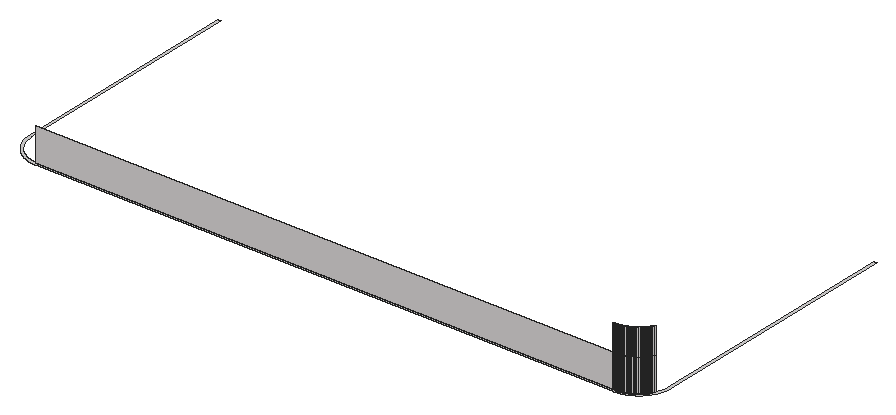
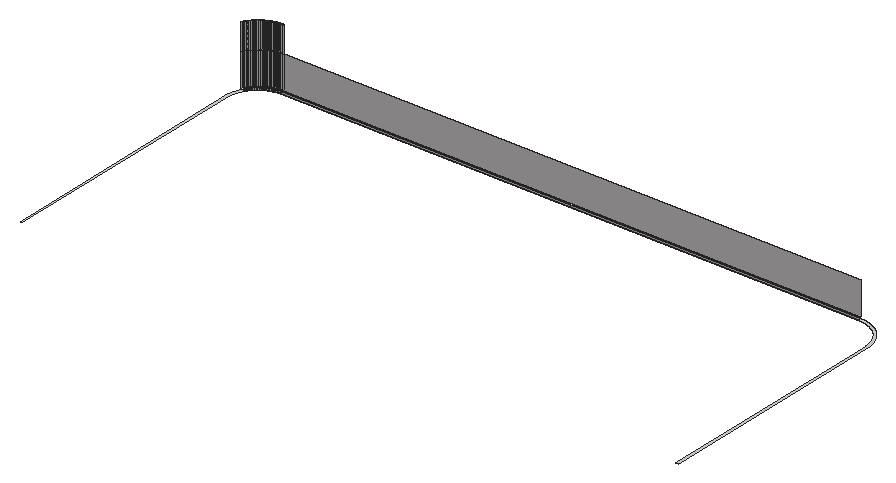
# SketchUp Ruby script. Lengths in inches.
U = 1.inch
M = Sketchup.active_model
def pt(a) = Geom::Point3d.new(a.map { |v| v * U })
def face(e, loops, mat)
  f = e.add_face(loops[0].map { |a| pt(a) })
  loops[1..].each { |l| e.add_face(l.map { |a| pt(a) }).erase! }
  f.material = f.back_material = mat if mat
  f
end
# faces: each face lists its corners as indices into pts; further lists are holes
def faces(e, pts, list, mat = nil) = list.each { |f| face(e, (f[0].is_a?(Array) ? f : [f]).map { |l| l.map { |i| pts[i] } }, mat) }
# xy, xz, yz: faces in a plane at the given z, y or x. An outline is a flat list of corners, or four numbers for a rectangle; further outlines are holes
def ring(l) = l.size == 4 ? [[l[0], l[1]], [l[2], l[1]], [l[2], l[3]], [l[0], l[3]]] : l.each_slice(2).to_a
def flat(e, list, mat, &to3) = list.each { |f| face(e, (f[0].is_a?(Array) ? f : [f]).map { |l| ring(l).map { |u, v| to3.(u, v) } }, mat) }
def xy(e, z, list, mat = nil) = flat(e, list, mat) { |x, y| [x, y, z] }
def xz(e, y, list, mat = nil) = flat(e, list, mat) { |x, z| [x, y, z] }
def yz(e, x, list, mat = nil) = flat(e, list, mat) { |y, z| [x, y, z] }
def lines(e, pts, list) = list.each { |a, b| e.add_line(pt(pts[a]), pt(pts[b])) }
# prism: a flat outline (further loops are holes) pulled along v
def prism(e, loops, v, mat = nil)
  f = face(e, loops, mat); d = Geom::Vector3d.new(v.map { |x| x * U })
  f.pushpull(f.normal.samedirection?(d) ? d.length : -d.length)
end
def box(e, o, s, mat = nil) = prism(e, [[o, [o[0] + s[0], o[1], o[2]], [o[0] + s[0], o[1] + s[1], o[2]], [o[0], o[1] + s[1], o[2]]]], [0, 0, s[2]], mat)
def at(x, y, z, deg = 0) = Geom::Transformation.translation(pt([x, y, z])) * Geom::Transformation.rotation(ORIGIN, Z_AXIS, deg.degrees)
def axes(o, x, y, z) = Geom::Transformation.new([*x, 0, *y, 0, *z, 0, *pt(o).to_a, 1])
def part(name) = M.definitions.add(name)
# library, detail: a bought-in or finely detailed component or shape, given as its bounding box
def library(name, o, s) = part(name).tap { |d| box(d.entities, o, s) }
def detail(e, o, s) = box(e.add_group.entities, o, s)
def put(e, d, t, mat = nil) = e.add_instance(d, t).tap { |i| i.material = mat if mat }
def group(e, t, mat = nil) = e.add_group.tap { |g| g.transformation = t; g.material = mat if mat }.entities
root = M.entities
M.materials.add("[Quartz Light Brown]").color = [215, 212, 212]
xy(root,368,[[215.8,143,480.2,143,480.39,143.01,480.59,143.01,480.79,143.02,480.98,143.03,481.18,143.05,481.37,143.0625,481.57,143.08,481.76,143.1,481.96,143.13,482.15,143.16,482.35,143.18,482.54,143.22,482.73,143.25,482.93,143.29,483.5,143.41,483.88,143.51,484.07,143.5625,484.26,143.62,484.45,143.67,484.64,143.73,484.82,143.8,485.01,143.86,485.19,143.93,485.56,144.07,485.74,144.14,486.46,144.46,486.63,144.55,486.81,144.63,486.98,144.73,487.16,144.82,487.33,144.91,487.84,145.21,488,145.3125,488.17,145.42,488.33,145.53,488.5,145.64,488.82,145.86,488.97,145.98,489.29,146.22,489.44,146.34,489.59,146.47,489.74,146.59,490.04,146.85,490.18,146.99,490.33,147.12,490.47,147.26,490.61,147.39,490.74,147.53,490.88,147.67,491.01,147.82,491.15,147.96,491.41,148.26,491.53,148.41,491.66,148.56,491.78,148.71,492.02,149.03,492.14,149.18,492.36,149.5,492.47,149.67,492.58,149.83,492.6875,150,492.79,150.16,493.09,150.67,493.18,150.84,493.27,151.02,493.37,151.19,493.45,151.37,493.54,151.54,493.86,152.26,493.93,152.44,494.07,152.81,494.14,152.99,494.2,153.18,494.27,153.36,494.33,153.55,494.38,153.74,494.4375,153.93,494.49,154.12,494.59,154.5,494.71,155.07,494.75,155.27,494.78,155.46,494.82,155.65,494.84,155.85,494.87,156.04,494.9,156.24,494.92,156.43,494.9375,156.63,494.95,156.82,494.97,157.02,494.98,157.21,494.99,157.41,494.99,157.61,495,157.8,495,275,494,275,494,157.63,493.98,157.27,493.97,157.08,493.96,156.9,493.92,156.54,493.9,156.35,493.86,155.99,493.77,155.45,493.57,154.55,493.47,154.2,493.42,154.02,493.37,153.85,493.31,153.67,493.26,153.5,493.2,153.33,493.13,153.15,493.07,152.98,493,152.8125,492.93,152.64,492.86,152.47,492.79,152.31,492.71,152.14,492.64,151.97,492.56,151.81,492.47,151.64,492.39,151.48,492.21,151.16,492.125,151,492.03,150.84,491.9375,150.69,491.84,150.53,491.64,150.22,491.54,150.07,491.43,149.92,491.33,149.77,491.11,149.48,490.99,149.33,490.88,149.19,490.76,149.05,490.65,148.91,490.53,148.77,490.4,148.63,490.28,148.5,490.16,148.36,489.64,147.84,489.5,147.72,489.37,147.6,489.23,147.47,489.09,147.35,488.95,147.24,488.81,147.12,488.67,147.01,488.52,146.89,488.23,146.67,488.08,146.57,487.93,146.46,487.78,146.36,487.47,146.16,487.31,146.0625,487.16,145.97,487,145.875,486.84,145.79,486.52,145.61,486.36,145.53,486.19,145.44,486.03,145.36,485.86,145.29,485.69,145.21,485.53,145.14,485.36,145.07,485.1875,145,485.02,144.93,484.85,144.87,484.67,144.8,484.5,144.74,484.33,144.69,484.15,144.63,483.98,144.58,483.8,144.53,483.45,144.43,482.55,144.23,482.01,144.14,481.65,144.1,481.46,144.08,481.1,144.04,480.92,144.03,480.73,144.02,480.37,144,215.63,144,215.27,144.02,215.08,144.03,214.9,144.04,214.54,144.08,214.35,144.1,213.99,144.14,213.45,144.23,212.55,144.43,212.2,144.53,212.02,144.58,211.85,144.63,211.67,144.69,211.5,144.74,211.33,144.8,211.15,144.87,210.98,144.93,210.8125,145,210.64,145.07,210.47,145.14,210.31,145.21,210.14,145.29,209.97,145.36,209.81,145.44,209.64,145.53,209.48,145.61,209.16,145.79,209,145.875,208.84,145.97,208.69,146.0625,208.53,146.16,208.22,146.36,208.07,146.46,207.92,146.57,207.77,146.67,207.48,146.89,207.33,147.01,207.19,147.12,207.05,147.24,206.91,147.35,206.77,147.47,206.63,147.6,206.5,147.72,206.36,147.84,205.84,148.36,205.72,148.5,205.6,148.63,205.47,148.77,205.35,148.91,205.24,149.05,205.12,149.19,205.01,149.33,204.89,149.48,204.67,149.77,204.57,149.92,204.46,150.07,204.36,150.22,204.16,150.53,204.0625,150.69,203.97,150.84,203.875,151,203.79,151.16,203.61,151.48,203.53,151.64,203.44,151.81,203.36,151.97,203.29,152.14,203.21,152.31,203.14,152.47,203.07,152.64,203,152.8125,202.93,152.98,202.87,153.15,202.8,153.33,202.74,153.5,202.69,153.67,202.63,153.85,202.58,154.02,202.53,154.2,202.43,154.55,202.23,155.45,202.14,155.99,202.1,156.35,202.08,156.54,202.04,156.9,202.03,157.08,202.02,157.27,202,157.63,202,266,201,266,201,157.8,201.01,157.61,201.01,157.41,201.02,157.21,201.03,157.02,201.05,156.82,201.0625,156.63,201.08,156.43,201.1,156.24,201.13,156.04,201.16,155.85,201.18,155.65,201.22,155.46,201.25,155.27,201.29,155.07,201.41,154.5,201.51,154.12,201.5625,153.93,201.62,153.74,201.67,153.55,201.73,153.36,201.8,153.18,201.86,152.99,201.93,152.81,202.07,152.44,202.14,152.26,202.46,151.54,202.55,151.37,202.63,151.19,202.73,151.02,202.82,150.84,202.91,150.67,203.21,150.16,203.3125,150,203.42,149.83,203.53,149.67,203.64,149.5,203.86,149.18,203.98,149.03,204.22,148.71,204.34,148.56,204.47,148.41,204.59,148.26,204.85,147.96,204.99,147.82,205.12,147.67,205.26,147.53,205.39,147.39,205.53,147.26,205.67,147.12,205.82,146.99,205.96,146.85,206.26,146.59,206.41,146.47,206.56,146.34,206.71,146.22,207.03,145.98,207.18,145.86,207.5,145.64,207.67,145.53,207.83,145.42,208,145.3125,208.16,145.21,208.67,144.91,208.84,144.82,209.02,144.73,209.19,144.63,209.37,144.55,209.54,144.46,210.26,144.14,210.44,144.07,210.81,143.93,210.99,143.86,211.18,143.8,211.36,143.73,211.55,143.67,211.74,143.62,211.93,143.5625,212.12,143.51,212.5,143.41,213.07,143.29,213.27,143.25,213.46,143.22,213.65,143.18,213.85,143.16,214.04,143.13,214.24,143.1,214.43,143.08,214.63,143.0625,214.82,143.05,215.02,143.03,215.21,143.02,215.41,143.01,215.61,143.01]],"[Quartz Light Brown]")
xz(root,143,[[216,369,480,384],[480,369,480.2,384],[480,384,480.2,396]],"[Quartz Light Brown]")
xz(root,143.01,[[480.39,369,480.59,384],[480.39,384,480.59,396]],"[Quartz Light Brown]")
xz(root,144,[[216,368,480,369],[480,368,480.18,369],[480.18,368,480.37,369]],"[Quartz Light Brown]")
p = [[480.37,144,369],[480.37,144,368],[480.55,144.01,368],[480.55,144.01,369],[480.73,144.02,368],[480.73,144.02,369],
  [480.92,144.03,368],[480.92,144.03,369],[481.1,144.04,368],[481.1,144.04,369],[481.28,144.06,368],[481.28,144.06,369],
  [481.46,144.08,368],[481.46,144.08,369],[481.65,144.1,368],[481.65,144.1,369],[481.83,144.12,368],[481.83,144.12,369],
  [482.01,144.14,368],[482.01,144.14,369],[482.19,144.17,368],[482.19,144.17,369],[482.37,144.2,368],[482.37,144.2,369],
  [482.55,144.23,368],[482.55,144.23,369],[482.73,144.27,368],[482.73,144.27,369],[482.91,144.31,368],[482.91,144.31,369],
  [483.09,144.35,368],[483.09,144.35,369],[483.27,144.39,368],[483.27,144.39,369],[483.45,144.43,368],[483.45,144.43,369],
  [483.625,144.48,368],[483.625,144.48,369],[483.8,144.53,368],[483.8,144.53,369],[483.98,144.58,368],[483.98,144.58,369],
  [484.15,144.63,368],[484.15,144.63,369],[484.33,144.69,368],[484.33,144.69,369],[484.5,144.74,368],[484.5,144.74,369],
  [484.67,144.8,368],[484.67,144.8,369],[484.85,144.87,368],[484.85,144.87,369],[485.02,144.93,368],[485.02,144.93,369],
  [485.1875,145,368],[485.1875,145,369],[485.36,145.07,368],[485.36,145.07,369],[485.53,145.14,368],[485.53,145.14,369],
  [485.69,145.21,368],[485.69,145.21,369],[485.86,145.29,368],[485.86,145.29,369],[486.03,145.36,368],[486.03,145.36,369],
  [486.19,145.44,368],[486.19,145.44,369],[486.36,145.53,368],[486.36,145.53,369],[486.52,145.61,368],[486.52,145.61,369],
  [486.68,145.7,368],[486.68,145.7,369],[486.84,145.79,368],[486.84,145.79,369],[487,145.875,368],[487,145.875,369],
  [487.16,145.97,368],[487.16,145.97,369],[487.31,146.0625,368],[487.31,146.0625,369],[487.47,146.16,368],[487.47,146.16,369],
  [487.625,146.26,368],[487.625,146.26,369],[487.78,146.36,368],[487.78,146.36,369],[487.93,146.46,368],[487.93,146.46,369],
  [488.08,146.57,368],[488.08,146.57,369],[488.23,146.67,368],[488.23,146.67,369],[488.375,146.78,368],[488.375,146.78,369],
  [488.52,146.89,368],[488.52,146.89,369],[488.67,147.01,368],[488.67,147.01,369],[488.81,147.12,368],[488.81,147.12,369],
  [488.95,147.24,368],[488.95,147.24,369],[489.09,147.35,368],[489.09,147.35,369],[489.23,147.47,368],[489.23,147.47,369],
  [489.37,147.6,368],[489.37,147.6,369],[489.5,147.72,368],[489.5,147.72,369],[489.64,147.84,368],[489.64,147.84,369],
  [489.77,147.97,368],[489.77,147.97,369],[489.9,148.1,368],[489.9,148.1,369],[490.03,148.23,368],[490.03,148.23,369],
  [490.16,148.36,368],[490.16,148.36,369],[490.28,148.5,368],[490.28,148.5,369],[490.4,148.63,368],[490.4,148.63,369],
  [490.53,148.77,368],[490.53,148.77,369],[490.65,148.91,368],[490.65,148.91,369],[490.76,149.05,368],[490.76,149.05,369],
  [490.88,149.19,368],[490.88,149.19,369],[490.99,149.33,368],[490.99,149.33,369],[491.11,149.48,368],[491.11,149.48,369],
  [491.22,149.625,368],[491.22,149.625,369],[491.33,149.77,368],[491.33,149.77,369],[491.43,149.92,368],[491.43,149.92,369],
  [491.54,150.07,368],[491.54,150.07,369],[491.64,150.22,368],[491.64,150.22,369],[491.74,150.375,368],[491.74,150.375,369],
  [491.84,150.53,368],[491.84,150.53,369],[491.9375,150.69,368],[491.9375,150.69,369],[492.03,150.84,368],[492.03,150.84,369],
  [492.125,151,368],[492.125,151,369],[480.39,143.01,384],[480.2,143,384],[480.2,143,369],[480.39,143.01,369],
  [480.79,143.02,384],[480.59,143.01,384],[480.59,143.01,369],[480.79,143.02,369],[480.98,143.03,384],[480.98,143.03,369],
  [481.18,143.05,384],[481.18,143.05,369],[481.37,143.0625,384],[481.37,143.0625,369],[481.57,143.08,384],[481.57,143.08,369],
  [481.76,143.1,384],[481.76,143.1,369],[481.96,143.13,384],[481.96,143.13,369],[482.15,143.16,384],[482.15,143.16,369],
  [482.35,143.18,384],[482.35,143.18,369],[482.54,143.22,384],[482.54,143.22,369],[482.73,143.25,384],[482.73,143.25,369],
  [482.93,143.29,384],[482.93,143.29,369],[483.12,143.33,384],[483.12,143.33,369],[483.31,143.37,384],[483.31,143.37,369],
  [483.5,143.41,384],[483.5,143.41,369],[483.69,143.46,384],[483.69,143.46,369],[483.88,143.51,384],[483.88,143.51,369],
  [484.07,143.5625,384],[484.07,143.5625,369],[484.26,143.62,384],[484.26,143.62,369],[484.45,143.67,384],[484.45,143.67,369],
  [484.64,143.73,384],[484.64,143.73,369],[484.82,143.8,384],[484.82,143.8,369],[485.01,143.86,384],[485.01,143.86,369],
  [485.19,143.93,384],[485.19,143.93,369],[485.375,144,384],[485.375,144,369],[485.56,144.07,384],[485.56,144.07,369],
  [485.74,144.14,384],[485.74,144.14,369],[485.92,144.22,384],[485.92,144.22,369],[486.1,144.3,384],[486.1,144.3,369],
  [486.28,144.38,384],[486.28,144.38,369],[486.46,144.46,384],[486.46,144.46,369],[486.63,144.55,384],[486.63,144.55,369],
  [486.81,144.63,384],[486.81,144.63,369],[486.98,144.73,384],[486.98,144.73,369],[487.16,144.82,384],[487.16,144.82,369],
  [487.33,144.91,384],[487.33,144.91,369],[487.5,145.01,384],[487.5,145.01,369],[487.67,145.11,384],[487.67,145.11,369],
  [487.84,145.21,384],[487.84,145.21,369],[488,145.3125,384],[488,145.3125,369],[488.17,145.42,384],[488.17,145.42,369],
  [488.33,145.53,384],[488.33,145.53,369],[488.5,145.64,384],[488.5,145.64,369],[488.66,145.75,384],[488.66,145.75,369],
  [488.82,145.86,384],[488.82,145.86,369],[488.97,145.98,384],[488.97,145.98,369],[489.13,146.1,384],[489.13,146.1,369],
  [489.29,146.22,384],[489.29,146.22,369],[489.44,146.34,384],[489.44,146.34,369],[489.59,146.47,384],[489.59,146.47,369],
  [489.74,146.59,384],[489.74,146.59,369],[489.89,146.72,384],[489.89,146.72,369],[490.04,146.85,384],[490.04,146.85,369],
  [490.18,146.99,384],[490.18,146.99,369],[490.33,147.12,384],[490.33,147.12,369],[490.47,147.26,384],[490.47,147.26,369],
  [490.61,147.39,384],[490.61,147.39,369],[490.74,147.53,384],[490.74,147.53,369],[490.88,147.67,384],[490.88,147.67,369],
  [491.01,147.82,384],[491.01,147.82,369],[491.15,147.96,384],[491.15,147.96,369],[491.28,148.11,384],[491.28,148.11,369],
  [491.41,148.26,384],[491.41,148.26,369],[491.53,148.41,384],[491.53,148.41,369],[491.66,148.56,384],[491.66,148.56,369],
  [491.78,148.71,384],[491.78,148.71,369],[491.9,148.87,384],[491.9,148.87,369],[492.02,149.03,384],[492.02,149.03,369],
  [492.14,149.18,384],[492.14,149.18,369],[492.25,149.34,384],[492.25,149.34,369],[492.36,149.5,384],[492.36,149.5,369],
  [492.47,149.67,384],[492.47,149.67,369],[492.58,149.83,384],[492.58,149.83,369],[492.6875,150,384],[492.6875,150,369],
  [492.79,150.16,384],[492.79,150.16,369],[492.89,150.33,384],[492.89,150.33,369],[492.99,150.5,384],[492.99,150.5,369],
  [493.09,150.67,384],[493.09,150.67,369],[493.18,150.84,384],[493.18,150.84,369],[480.2,143,384],[480.39,143.01,384],
  [480.39,143.01,396],[480.2,143,396],[480.59,143.01,384],[480.79,143.02,384],[480.79,143.02,396],[480.59,143.01,396],
  [480.98,143.03,384],[480.98,143.03,396],[481.18,143.05,384],[481.18,143.05,396],[481.37,143.0625,384],[481.37,143.0625,396],
  [481.57,143.08,384],[481.57,143.08,396],[481.76,143.1,384],[481.76,143.1,396],[481.96,143.13,384],[481.96,143.13,396],
  [482.15,143.16,384],[482.15,143.16,396],[482.35,143.18,384],[482.35,143.18,396],[482.54,143.22,384],[482.54,143.22,396],
  [482.73,143.25,384],[482.73,143.25,396],[482.93,143.29,384],[482.93,143.29,396],[483.12,143.33,384],[483.12,143.33,396],
  [483.31,143.37,384],[483.31,143.37,396],[483.5,143.41,384],[483.5,143.41,396],[483.69,143.46,384],[483.69,143.46,396],
  [483.88,143.51,384],[483.88,143.51,396],[484.07,143.5625,384],[484.07,143.5625,396],[484.26,143.62,384],[484.26,143.62,396],
  [484.45,143.67,384],[484.45,143.67,396],[484.64,143.73,384],[484.64,143.73,396],[484.82,143.8,384],[484.82,143.8,396],
  [485.01,143.86,384],[485.01,143.86,396],[485.19,143.93,384],[485.19,143.93,396],[485.375,144,384],[485.375,144,396],
  [485.56,144.07,384],[485.56,144.07,396],[485.74,144.14,384],[485.74,144.14,396],[485.92,144.22,384],[485.92,144.22,396],
  [486.1,144.3,384],[486.1,144.3,396],[486.28,144.38,384],[486.28,144.38,396],[486.46,144.46,384],[486.46,144.46,396],
  [486.63,144.55,384],[486.63,144.55,396],[486.81,144.63,384],[486.81,144.63,396],[486.98,144.73,384],[486.98,144.73,396],
  [487.16,144.82,384],[487.16,144.82,396],[487.33,144.91,384],[487.33,144.91,396],[487.5,145.01,384],[487.5,145.01,396],
  [487.67,145.11,384],[487.67,145.11,396],[487.84,145.21,384],[487.84,145.21,396],[488,145.3125,384],[488,145.3125,396],
  [488.17,145.42,384],[488.17,145.42,396],[488.33,145.53,384],[488.33,145.53,396],[488.5,145.64,384],[488.5,145.64,396],
  [488.66,145.75,384],[488.66,145.75,396],[488.82,145.86,384],[488.82,145.86,396],[488.97,145.98,384],[488.97,145.98,396],
  [489.13,146.1,384],[489.13,146.1,396],[489.29,146.22,384],[489.29,146.22,396],[489.44,146.34,384],[489.44,146.34,396],
  [489.59,146.47,384],[489.59,146.47,396],[489.74,146.59,384],[489.74,146.59,396],[489.89,146.72,384],[489.89,146.72,396],
  [490.04,146.85,384],[490.04,146.85,396],[490.18,146.99,384],[490.18,146.99,396],[490.33,147.12,384],[490.33,147.12,396],
  [490.47,147.26,384],[490.47,147.26,396],[490.61,147.39,384],[490.61,147.39,396],[490.74,147.53,384],[490.74,147.53,396],
  [490.88,147.67,384],[490.88,147.67,396],[491.01,147.82,384],[491.01,147.82,396],[491.15,147.96,384],[491.15,147.96,396],
  [491.28,148.11,384],[491.28,148.11,396],[491.41,148.26,384],[491.41,148.26,396],[491.53,148.41,384],[491.53,148.41,396],
  [491.66,148.56,384],[491.66,148.56,396],[491.78,148.71,384],[491.78,148.71,396],[491.9,148.87,384],[491.9,148.87,396],
  [492.02,149.03,384],[492.02,149.03,396],[492.14,149.18,384],[492.14,149.18,396],[492.25,149.34,384],[492.25,149.34,396],
  [492.36,149.5,384],[492.36,149.5,396],[492.47,149.67,384],[492.47,149.67,396],[492.58,149.83,384],[492.58,149.83,396],
  [492.6875,150,384],[492.6875,150,396],[492.79,150.16,384],[492.79,150.16,396],[492.89,150.33,384],[492.89,150.33,396],
  [492.99,150.5,384],[492.99,150.5,396],[493.09,150.67,384],[493.09,150.67,396],[493.18,150.84,384],[493.18,150.84,396]]
faces(root,p,[[0,1,2,3],[3,2,4,5],[5,4,6,7],[7,6,8,9],[9,8,10,11],[11,10,12,13],[13,12,14,15],[15,14,16,17],
  [17,16,18,19],[19,18,20,21],[21,20,22,23],[23,22,24,25],[25,24,26,27],[27,26,28,29],[29,28,30,31],[31,30,32,33],
  [33,32,34,35],[35,34,36,37],[37,36,38,39],[39,38,40,41],[41,40,42,43],[43,42,44,45],[45,44,46,47],[47,46,48,49],
  [49,48,50,51],[51,50,52,53],[53,52,54,55],[55,54,56,57],[57,56,58,59],[59,58,60,61],[61,60,62,63],[63,62,64,65],
  [65,64,66,67],[67,66,68,69],[69,68,70,71],[71,70,72,73],[73,72,74,75],[75,74,76,77],[77,76,78,79],[79,78,80,81],
  [81,80,82,83],[83,82,84,85],[85,84,86,87],[87,86,88,89],[89,88,90,91],[91,90,92,93],[93,92,94,95],[95,94,96,97],
  [97,96,98,99],[99,98,100,101],[101,100,102,103],[103,102,104,105],[105,104,106,107],[107,106,108,109],[109,108,110,111],[111,110,112,113],
  [113,112,114,115],[115,114,116,117],[117,116,118,119],[119,118,120,121],[121,120,122,123],[123,122,124,125],[125,124,126,127],[127,126,128,129],
  [129,128,130,131],[131,130,132,133],[133,132,134,135],[135,134,136,137],[137,136,138,139],[139,138,140,141],[141,140,142,143],[143,142,144,145],
  [145,144,146,147],[147,146,148,149],[149,148,150,151],[151,150,152,153],[153,152,154,155],[155,154,156,157],[158,159,160,161],[162,163,164,165],
  [166,162,165,167],[168,166,167,169],[170,168,169,171],[172,170,171,173],[174,172,173,175],[176,174,175,177],[178,176,177,179],[180,178,179,181],
  [182,180,181,183],[184,182,183,185],[186,184,185,187],[188,186,187,189],[190,188,189,191],[192,190,191,193],[194,192,193,195],[196,194,195,197],
  [198,196,197,199],[200,198,199,201],[202,200,201,203],[204,202,203,205],[206,204,205,207],[208,206,207,209],[210,208,209,211],[212,210,211,213],
  [214,212,213,215],[216,214,215,217],[218,216,217,219],[220,218,219,221],[222,220,221,223],[224,222,223,225],[226,224,225,227],[228,226,227,229],
  [230,228,229,231],[232,230,231,233],[234,232,233,235],[236,234,235,237],[238,236,237,239],[240,238,239,241],[242,240,241,243],[244,242,243,245],
  [246,244,245,247],[248,246,247,249],[250,248,249,251],[252,250,251,253],[254,252,253,255],[256,254,255,257],[258,256,257,259],[260,258,259,261],
  [262,260,261,263],[264,262,263,265],[266,264,265,267],[268,266,267,269],[270,268,269,271],[272,270,271,273],[274,272,273,275],[276,274,275,277],
  [278,276,277,279],[280,278,279,281],[282,280,281,283],[284,282,283,285],[286,284,285,287],[288,286,287,289],[290,288,289,291],[292,290,291,293],
  [294,292,293,295],[296,294,295,297],[298,296,297,299],[300,298,299,301],[302,300,301,303],[304,302,303,305],[306,304,305,307],[308,306,307,309],
  [310,308,309,311],[312,310,311,313],[314,312,313,315],[316,314,315,317],[318,316,317,319],[320,318,319,321],[322,323,324,325],[326,327,328,329],
  [327,330,331,328],[330,332,333,331],[332,334,335,333],[334,336,337,335],[336,338,339,337],[338,340,341,339],[340,342,343,341],[342,344,345,343],
  [344,346,347,345],[346,348,349,347],[348,350,351,349],[350,352,353,351],[352,354,355,353],[354,356,357,355],[356,358,359,357],[358,360,361,359],
  [360,362,363,361],[362,364,365,363],[364,366,367,365],[366,368,369,367],[368,370,371,369],[370,372,373,371],[372,374,375,373],[374,376,377,375],
  [376,378,379,377],[378,380,381,379],[380,382,383,381],[382,384,385,383],[384,386,387,385],[386,388,389,387],[388,390,391,389],[390,392,393,391],
  [392,394,395,393],[394,396,397,395],[396,398,399,397],[398,400,401,399],[400,402,403,401],[402,404,405,403],[404,406,407,405],[406,408,409,407],
  [408,410,411,409],[410,412,413,411],[412,414,415,413],[414,416,417,415],[416,418,419,417],[418,420,421,419],[420,422,423,421],[422,424,425,423],
  [424,426,427,425],[426,428,429,427],[428,430,431,429],[430,432,433,431],[432,434,435,433],[434,436,437,435],[436,438,439,437],[438,440,441,439],
  [440,442,443,441],[442,444,445,443],[444,446,447,445],[446,448,449,447],[448,450,451,449],[450,452,453,451],[452,454,455,453],[454,456,457,455],
  [456,458,459,457],[458,460,461,459],[460,462,463,461],[462,464,465,463],[464,466,467,465],[466,468,469,467],[468,470,471,469],[470,472,473,471],
  [472,474,475,473],[474,476,477,475],[476,478,479,477],[478,480,481,479],[480,482,483,481],[482,484,485,483]],"[Quartz Light Brown]")
